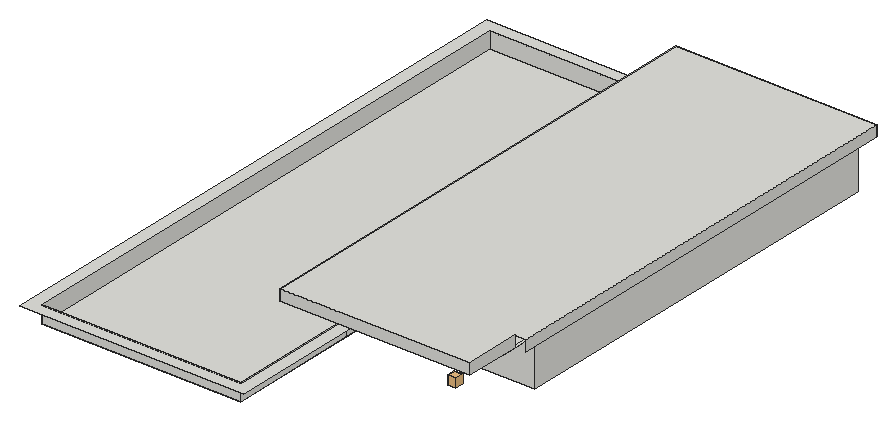
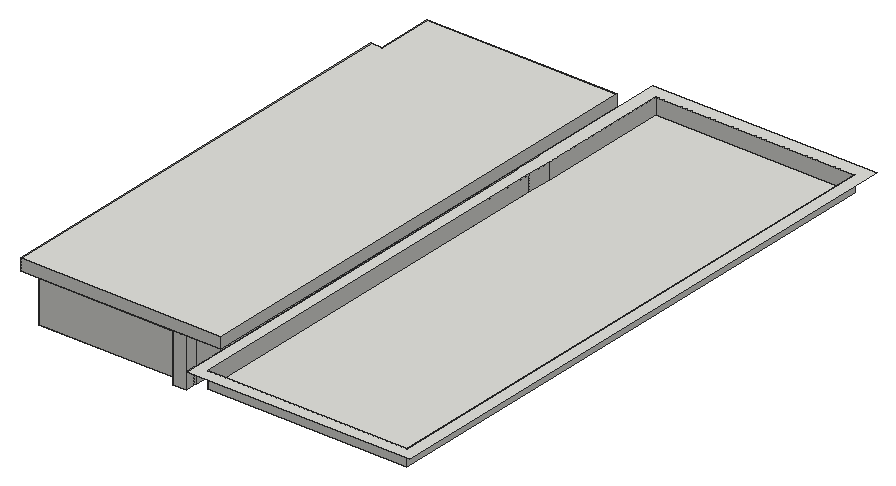
# SketchUp Ruby script. Lengths in inches.
U = 1.inch
M = Sketchup.active_model
def pt(a) = Geom::Point3d.new(a.map { |v| v * U })
def face(e, loops, mat)
  f = e.add_face(loops[0].map { |a| pt(a) })
  loops[1..].each { |l| e.add_face(l.map { |a| pt(a) }).erase! }
  f.material = f.back_material = mat if mat
  f
end
# faces: each face lists its corners as indices into pts; further lists are holes
def faces(e, pts, list, mat = nil) = list.each { |f| face(e, (f[0].is_a?(Array) ? f : [f]).map { |l| l.map { |i| pts[i] } }, mat) }
# xy, xz, yz: faces in a plane at the given z, y or x. An outline is a flat list of corners, or four numbers for a rectangle; further outlines are holes
def ring(l) = l.size == 4 ? [[l[0], l[1]], [l[2], l[1]], [l[2], l[3]], [l[0], l[3]]] : l.each_slice(2).to_a
def flat(e, list, mat, &to3) = list.each { |f| face(e, (f[0].is_a?(Array) ? f : [f]).map { |l| ring(l).map { |u, v| to3.(u, v) } }, mat) }
def xy(e, z, list, mat = nil) = flat(e, list, mat) { |x, y| [x, y, z] }
def xz(e, y, list, mat = nil) = flat(e, list, mat) { |x, z| [x, y, z] }
def yz(e, x, list, mat = nil) = flat(e, list, mat) { |y, z| [x, y, z] }
def lines(e, pts, list) = list.each { |a, b| e.add_line(pt(pts[a]), pt(pts[b])) }
# prism: a flat outline (further loops are holes) pulled along v
def prism(e, loops, v, mat = nil)
  f = face(e, loops, mat); d = Geom::Vector3d.new(v.map { |x| x * U })
  f.pushpull(f.normal.samedirection?(d) ? d.length : -d.length)
end
def box(e, o, s, mat = nil) = prism(e, [[o, [o[0] + s[0], o[1], o[2]], [o[0] + s[0], o[1] + s[1], o[2]], [o[0], o[1] + s[1], o[2]]]], [0, 0, s[2]], mat)
def at(x, y, z, deg = 0) = Geom::Transformation.translation(pt([x, y, z])) * Geom::Transformation.rotation(ORIGIN, Z_AXIS, deg.degrees)
def axes(o, x, y, z) = Geom::Transformation.new([*x, 0, *y, 0, *z, 0, *pt(o).to_a, 1])
def part(name) = M.definitions.add(name)
# library, detail: a bought-in or finely detailed component or shape, given as its bounding box
def library(name, o, s) = part(name).tap { |d| box(d.entities, o, s) }
def detail(e, o, s) = box(e.add_group.entities, o, s)
def put(e, d, t, mat = nil) = e.add_instance(d, t).tap { |i| i.material = mat if mat }
def group(e, t, mat = nil) = e.add_group.tap { |g| g.transformation = t; g.material = mat if mat }.entities
root = M.entities
M.materials.add("Glass_Tinted_Gray").color = [0, 0, 0]
M.materials["Glass_Tinted_Gray"].alpha = 0.125
M.materials.add("[0135_DarkGray]").color = [81, 81, 81]
M.materials.add("[Mirror 02]").color = [229, 229, 229]
M.materials.add("[Terrazzo Light Blue]").color = [196, 214, 227]
M.materials.add("[Wood Veneer 01]").color = [120, 70, 37]
c1 = library("Spot Light",[-5.1,-5.1,-11.05],[10.2,10.2,11.05])
c2 = part("PENTEK_RP Fineline 50S_Sliding_DoorCase_E1")
box(c2.entities,[0,0,0],[1.51,3.66,99.27],"[0135_DarkGray]")
c3 = part("PENTEK_RP Fineline 50S_SlidingDooe_Case_E2")
box(c3.entities,[0,0,0],[96.25,3.66,1.51],"[0135_DarkGray]")
c4 = part("pentek_RP Fineline 50S_SlidingDoor_Case")
put(c4.entities,c2,at(97.76,0,0))
put(c4.entities,c3,at(1.51,0,0))
put(c4.entities,c2,at(0,0,0))
put(c4.entities,c3,at(1.51,0,97.76))
c5 = part("PENTEK_RP Fineline 50S_SlidingDoor_GlazingBead_2")
box(c5.entities,[0,0,0],[0.56,0.59,94.39],"[0135_DarkGray]")
c6 = part("PENTEK_RP Fineline 50S_SlidingDoor_Glass")
box(c6.entities,[0,0,0],[46.58,0.16,94.39],"Glass_Tinted_Gray")
c7 = part("PENTEK_RP Fineline 50S_SlidingDoor_GlazingBead")
box(c7.entities,[0,0,0],[45.47,0.59,0.56],"[0135_DarkGray]")
c8 = part("PENTEK_RP Fineline 50S_SlidingDoor_Leaf_E1")
xy(c8.entities,0,[[0,0,0.93,1.97],[0.93,1.57,1.49,1.97]],"[0135_DarkGray]")
xy(c8.entities,96.25,[[0,0,0.93,0,0.93,1.57,1.49,1.57,1.49,1.97,0,1.97]],"[0135_DarkGray]")
xz(c8.entities,0,[[0,0,0.93,96.25]],"[0135_DarkGray]")
xz(c8.entities,1.57,[[0.93,0,1.49,95.32],[0.93,95.32,1.49,96.25]],"[0135_DarkGray]")
xz(c8.entities,1.97,[[0,0,1.49,96.25]],"[0135_DarkGray]")
yz(c8.entities,0,[[0,0,1.97,96.25]],"[0135_DarkGray]")
yz(c8.entities,0.93,[[0,0,1.57,0.93],[0,0.93,1.57,95.32],[0,95.32,1.57,96.25]],"[0135_DarkGray]")
yz(c8.entities,1.49,[[1.57,0,1.97,95.32],[1.57,95.32,1.97,96.25]],"[0135_DarkGray]")
c9 = part("PENTEK_RP Fineline 50S_SlidingDoor_Leaf_E2")
xy(c9.entities,0,[[0,0,0,1.57,0.56,1.57,0.56,1.97,46.02,1.97,46.02,1.57,46.58,1.57,46.58,0]],"[0135_DarkGray]")
xy(c9.entities,0.93,[[0,0,46.58,1.57]],"[0135_DarkGray]")
xy(c9.entities,1.49,[[0.56,1.57,46.02,1.97]],"[0135_DarkGray]")
xz(c9.entities,0,[[0,0,46.58,0.93]],"[0135_DarkGray]")
xz(c9.entities,1.57,[[0,0,0.56,0.93],[46.02,0,46.58,0.93],[0.56,0.93,46.02,1.49]],"[0135_DarkGray]")
xz(c9.entities,1.97,[[0.56,0,46.02,1.49]],"[0135_DarkGray]")
yz(c9.entities,0,[[0,0,1.57,0.93]],"[0135_DarkGray]")
yz(c9.entities,0.56,[[1.57,0,1.97,0.93],[1.57,0.93,1.97,1.49]],"[0135_DarkGray]")
yz(c9.entities,46.02,[[1.57,0,1.97,0.93],[1.57,0.93,1.97,1.49]],"[0135_DarkGray]")
yz(c9.entities,46.58,[[0,0,1.57,0.93]],"[0135_DarkGray]")
c10 = part("PENTEK_RP Fineline S_SlidingDoor_Leaf1")
put(c10.entities,c5,at(0.93,0,0.93))
put(c10.entities,c5,at(46.96,0,0.93))
put(c10.entities,c6,at(1.49,1.42,0.93))
put(c10.entities,c7,at(1.49,0,0.93))
put(c10.entities,c6,at(1.49,0.59,0.93),"[Terrazzo Light Blue]")
put(c10.entities,c8,at(0,0,0))
put(c10.entities,c8,axes([48.44,0,0],[-1,0,0],[0,1,0],[0,0,1]))
put(c10.entities,c9,axes([0.93,0,96.25],[1,0,0],[0,1,0],[0,0,-1]))
put(c10.entities,c9,at(0.93,0,0))
put(c10.entities,c7,at(1.49,0,94.77))
c11 = part("PENTEK_RP Fineline 50S_SlidingDoor_Leaf2")
put(c11.entities,c6,at(1.49,1.42,0.93))
put(c11.entities,c7,at(1.49,0,94.77))
put(c11.entities,c5,at(46.96,0,0.93))
put(c11.entities,c6,at(1.49,0.59,0.93),"[Mirror 02]")
put(c11.entities,c5,at(0.93,0,0.93))
put(c11.entities,c8,at(0,0,0))
put(c11.entities,c8,axes([48.44,0,0],[-1,0,0],[0,1,0],[0,0,1]))
put(c11.entities,c7,at(1.49,0,0.93))
put(c11.entities,c9,axes([0.93,0,96.25],[1,0,0],[0,1,0],[0,0,-1]))
put(c11.entities,c9,at(0.93,0,0))
c12 = part("PENTEK - Slimmest Steel Sliding Door / Window\#1")
put(c12.entities,c4,at(0,-1.88,-0.09))
put(c12.entities,c10,at(1.51,-2.27,1.42))
put(c12.entities,c11,at(49.32,-0.3,1.42))
c13 = part("Group76\#1")
p = [[0,0,0],[0,0,-13.3125],[-1.22,0,-13.3125],[7.92,-35.18,0],[-7.92,-35.18,0],[7.92,35.18,0],
  [7.92,0,0],[-7.92,35.18,0],[1.22,0,-13.3125],[-7.92,0,0],[0,0,-21.55]]
lines(c13.entities,p,[[0,1],[1,2],[3,4],[5,6],[7,5],[1,8],[9,0],[0,6],[8,10],[4,9],[6,3],[2,10],
  [9,7]])
c14 = part("Rectangle Light\#2")
put(c14.entities,c13,at(0,0,0))
c15 = library("Group\#24",[-0.5,-0.5,0],[156.52,11,0.25])
xy(root,379.1875,[[223.8125,438.06,222.26,438.25,220.8125,438.85,219.5625,439.8,218.61,441.04,218,442.48,217.79,444.03,217.99,445.59,218.58,447.04,219.53,448.28,220.77,449.24,222.22,449.84,223.77,450.06,225.32,449.86,226.77,449.26,228.02,448.3125,228.98,447.08,229.58,445.63,229.79,444.08,229.59,442.52,229,441.08,228.05,439.83,226.81,438.87,225.37,438.27],[274.1875,438.06,272.63,438.25,271.1875,438.85,269.9375,439.8,268.98,441.04,268.375,442.48,268.17,444.03,268.36,445.59,268.96,447.04,269.91,448.28,271.15,449.24,272.59,449.84,274.14,450.06,275.7,449.86,277.15,449.26,278.39,448.3125,279.35,447.08,279.96,445.63,280.17,444.08,279.97,442.52,279.375,441.08,278.42,439.83,277.19,438.87,275.74,438.27],[322.8125,438.06,321.26,438.25,319.8125,438.85,318.5625,439.8,317.61,441.04,317,442.48,316.79,444.03,316.99,445.59,317.58,447.04,318.53,448.28,319.77,449.24,321.22,449.84,322.77,450.06,324.32,449.86,325.77,449.26,327.02,448.3125,327.98,447.08,328.58,445.63,328.79,444.08,328.59,442.52,328,441.08,327.05,439.83,325.81,438.87,324.37,438.27],[388.8125,438.06,387.26,438.25,385.8125,438.85,384.5625,439.8,383.61,441.04,383,442.48,382.79,444.03,382.99,445.59,383.58,447.04,384.53,448.28,385.77,449.24,387.22,449.84,388.77,450.06,390.32,449.86,391.77,449.26,393.02,448.3125,393.98,447.08,394.58,445.63,394.79,444.08,394.59,442.52,394,441.08,393.05,439.83,391.81,438.87,390.37,438.27],[223.79,540.64,222.24,540.85,220.79,541.45,219.55,542.4,218.59,543.64,217.99,545.09,217.79,546.64,217.99,548.2,218.59,549.64,219.55,550.89,220.79,551.84,222.24,552.4375,223.79,552.64,225.34,552.4375,226.79,551.84,228.03,550.89,228.99,549.64,229.59,548.2,229.79,546.64,229.59,545.09,228.99,543.64,228.03,542.4,226.79,541.45,225.34,540.85],
  [274.17,540.64,272.61,540.85,271.17,541.45,269.92,542.4,268.97,543.64,268.37,545.09,268.17,546.64,268.37,548.2,268.97,549.64,269.92,550.89,271.17,551.84,272.61,552.4375,274.17,552.64,275.72,552.4375,277.17,551.84,278.41,550.89,279.36,549.64,279.96,548.2,280.17,546.64,279.96,545.09,279.36,543.64,278.41,542.4,277.17,541.45,275.72,540.85],[322.79,540.64,321.24,540.85,319.79,541.45,318.55,542.4,317.59,543.64,316.99,545.09,316.79,546.64,316.99,548.2,317.59,549.64,318.55,550.89,319.79,551.84,321.24,552.4375,322.79,552.64,324.34,552.4375,325.79,551.84,327.03,550.89,327.99,549.64,328.59,548.2,328.79,546.64,328.59,545.09,327.99,543.64,327.03,542.4,325.79,541.45,324.34,540.85],[388.79,540.64,387.24,540.85,385.79,541.45,384.55,542.4,383.59,543.64,382.99,545.09,382.79,546.64,382.99,548.2,383.59,549.64,384.55,550.89,385.79,551.84,387.24,552.4375,388.79,552.64,390.34,552.4375,391.79,551.84,393.03,550.89,393.99,549.64,394.59,548.2,394.79,546.64,394.59,545.09,393.99,543.64,393.03,542.4,391.79,541.45,390.34,540.85]])
xy(root,381.03,[[572.68,554.8125,578.99,562.125]])
xy(root,384,[[192.6,398.16,438.02,1088.46],[452.87,593.61,469.06,1087.125],[469.06,593.61,469.08,1091.4],[469.08,593.61,644.41,1091.4],[452.87,1087.125,469.06,1091.4],
  [452.87,1091.4,469.06,1103.3125]])
xy(root,404.125,[[[177.75,383.3125,452.87,1103.3125],[192.6,398.16,438.02,1088.46]]])
xy(root,408.9,[[484.27,562.125,554.02,593.61]])
xy(root,429.22,[[484.27,562.125,554.02,593.61]])
xy(root,431.7,[[597.99,562.125,631.02,589.625]])
xy(root,444,[[452.87,562.125,469.06,593.61],[469.06,562.125,641.5625,593.61],[641.5625,562.125,644.41,593.61],[452.87,593.61,469.06,1087.125],[469.06,593.61,641.5625,1087.125],
  [641.5625,593.61,644.41,1087.125],[452.87,1087.125,469.06,1103.3125],[469.06,1087.125,644.41,1091.4],[644.41,1087.125,657.75,1103.3125],[469.06,1091.4,644.41,1103.3125]])
xy(root,444,[[[410.81,492.5,410.81,1103.3125,452.87,1103.3125,452.87,562.125,644.41,562.125,644.41,492.5],[577.39,512.37,578.68,512.54,579.89,513.04,580.93,513.84,581.72,514.87,582.22,516.08,582.39,517.37,582.22,518.67,581.72,519.87,580.93,520.91,579.89,521.7,578.68,522.2,577.39,522.37,576.1,522.2,574.89,521.7,573.86,520.91,573.06,519.87,572.5625,518.67,572.39,517.37,572.5625,516.08,573.06,514.87,573.86,513.84,574.89,513.04,576.1,512.54],[470.07,512.37,471.37,512.54,472.57,513.04,473.61,513.84,474.4,514.87,474.9,516.08,475.07,517.37,474.9,518.67,474.4,519.87,473.61,520.91,472.57,521.7,471.37,522.2,470.07,522.37,468.78,522.2,467.57,521.7,466.54,520.91,465.74,519.87,465.24,518.67,465.07,517.37,465.24,516.08,465.74,514.87,466.54,513.84,467.57,513.04,468.78,512.54],[527.61,513.44,528.625,513.57,529.58,513.96,530.39,514.59,531.02,515.4,531.41,516.35,531.54,517.37,531.41,518.39,531.02,519.34,530.39,520.16,529.58,520.78,528.625,521.18,527.61,521.31,526.59,521.18,525.64,520.78,524.82,520.16,524.2,519.34,523.8,518.39,523.67,517.37,523.8,516.35,524.2,515.4,524.82,514.59,525.64,513.96,526.59,513.57],[616.93,513.71,617.88,513.83,618.76,514.2,619.52,514.78,620.1,515.54,620.47,516.42,620.59,517.37,620.47,518.32,620.1,519.2,619.52,519.96,618.76,520.55,617.88,520.91,616.93,521.04,615.98,520.91,615.1,520.55,614.34,519.96,613.76,519.2,613.39,518.32,613.27,517.37,613.39,516.42,613.76,515.54,614.34,514.78,615.1,514.2,615.98,513.83]]],"[Wood Veneer 01]")
xy(root,457.625,[[410.81,492.5,644.41,492.5,644.41,562.125,657.75,562.125,657.75,1103.3125,410.81,1103.3125]])
xz(root,398.16,[[192.6,384,438.02,404.125]])
xz(root,492.5,[[410.81,444,644.41,457.625]])
xz(root,593.61,[[452.87,384,469.06,444],[[469.06,384,644.41,444],[484.27,408.9,554.02,429.22]]])
xz(root,1087.125,[[452.87,384,469.06,444]])
xz(root,1088.46,[[192.6,384,438.02,404.125]])
xz(root,1091.4,[[469.06,384,644.41,444]])
xz(root,1103.3125,[[452.87,384,469.06,444],[410.81,444,657.75,457.625]])
yz(root,192.6,[[398.16,384,1088.46,404.125]])
yz(root,410.81,[[492.5,444,1103.3125,457.625]])
yz(root,438.02,[[398.16,384,562.125,404.125],[562.125,384,593.61,404.125],[593.61,384,1087.125,404.125],[1087.125,384,1088.46,404.125]])
yz(root,452.87,[[593.61,384,1087.125,404.125],[1087.125,384,1091.4,404.125],[1091.4,384,1103.3125,404.125],[562.125,404.125,593.61,444],[593.61,404.125,1087.125,444],
  [1087.125,404.125,1103.3125,444]])
yz(root,469.06,[[593.61,384,1087.125,444],[1087.125,384,1091.4,444],[1091.4,384,1103.3125,444]])
yz(root,484.27,[[562.125,408.9,593.61,429.22]])
yz(root,554.02,[[562.125,408.9,593.61,429.22]])
yz(root,644.41,[[593.61,384,1091.4,444],[492.5,444,562.125,457.625]])
yz(root,657.75,[[562.125,444,1103.3125,457.625]])
p = [[470.07,512.37,444],[468.78,512.54,444],[468.78,512.54,445.375],[470.07,512.37,445.375],[471.37,512.54,444],[471.37,512.54,445.375],
  [577.39,512.37,444],[576.1,512.54,444],[576.1,512.54,445.375],[577.39,512.37,445.375],[578.68,512.54,444],[578.68,512.54,445.375],
  [467.57,513.04,444],[467.57,513.04,445.375],[472.57,513.04,444],[472.57,513.04,445.375],[574.89,513.04,444],[574.89,513.04,445.375],
  [579.89,513.04,444],[579.89,513.04,445.375],[466.54,513.84,444],[466.54,513.84,445.375],[473.61,513.84,444],[473.61,513.84,445.375],
  [573.86,513.84,444],[573.86,513.84,445.375],[580.93,513.84,444],[580.93,513.84,445.375],[527.61,513.44,444],[526.59,513.57,444],
  [526.59,513.57,445.375],[527.61,513.44,445.375],[528.625,513.57,444],[528.625,513.57,445.375],[525.64,513.96,444],[525.64,513.96,445.375],
  [529.58,513.96,444],[529.58,513.96,445.375],[616.93,513.71,444],[615.98,513.83,444],[615.98,513.83,445.625],[616.93,513.71,445.625],
  [617.88,513.83,444],[617.88,513.83,445.625],[465.74,514.87,444],[465.74,514.87,445.375],[474.4,514.87,444],[474.4,514.87,445.375],
  [573.06,514.87,444],[573.06,514.87,445.375],[581.72,514.87,444],[581.72,514.87,445.375],[615.1,514.2,444],[615.1,514.2,445.625],
  [618.76,514.2,444],[618.76,514.2,445.625],[524.82,514.59,444],[524.82,514.59,445.375],[530.39,514.59,444],[530.39,514.59,445.375],
  [614.34,514.78,444],[614.34,514.78,445.625],[619.52,514.78,444],[619.52,514.78,445.625],[524.2,515.4,444],[524.2,515.4,445.375],
  [531.02,515.4,444],[531.02,515.4,445.375],[613.76,515.54,444],[613.76,515.54,445.625],[620.1,515.54,444],[620.1,515.54,445.625],
  [465.24,516.08,444],[465.24,516.08,445.375],[474.9,516.08,444],[474.9,516.08,445.375],[572.5625,516.08,444],[572.5625,516.08,445.375],
  [582.22,516.08,444],[582.22,516.08,445.375],[523.8,516.35,444],[523.8,516.35,445.375],[531.41,516.35,444],[531.41,516.35,445.375],
  [613.39,516.42,444],[613.39,516.42,445.625],[620.47,516.42,444],[620.47,516.42,445.625],[465.07,517.37,444],[465.07,517.37,445.375],
  [475.07,517.37,444],[475.07,517.37,445.375],[572.39,517.37,444],[572.39,517.37,445.375],[582.39,517.37,444],[582.39,517.37,445.375],
  [523.67,517.37,444],[523.67,517.37,445.375],[531.54,517.37,444],[531.54,517.37,445.375],[613.27,517.37,444],[613.27,517.37,445.625],
  [620.59,517.37,444],[620.59,517.37,445.625],[465.24,518.67,444],[465.24,518.67,445.375],[474.9,518.67,444],[474.9,518.67,445.375],
  [523.8,518.39,444],[523.8,518.39,445.375],[531.41,518.39,444],[531.41,518.39,445.375],[572.5625,518.67,444],[572.5625,518.67,445.375],
  [582.22,518.67,444],[582.22,518.67,445.375],[613.39,518.32,444],[613.39,518.32,445.625],[620.47,518.32,444],[620.47,518.32,445.625],
  [613.76,519.2,444],[613.76,519.2,445.625],[620.1,519.2,444],[620.1,519.2,445.625],[524.2,519.34,444],[524.2,519.34,445.375],
  [531.02,519.34,444],[531.02,519.34,445.375],[465.74,519.87,444],[465.74,519.87,445.375],[474.4,519.87,444],[474.4,519.87,445.375],
  [573.06,519.87,444],[573.06,519.87,445.375],[581.72,519.87,444],[581.72,519.87,445.375],[614.34,519.96,444],[614.34,519.96,445.625],
  [619.52,519.96,444],[619.52,519.96,445.625],[524.82,520.16,444],[524.82,520.16,445.375],[530.39,520.16,444],[530.39,520.16,445.375],
  [466.54,520.91,444],[466.54,520.91,445.375],[473.61,520.91,444],[473.61,520.91,445.375],[573.86,520.91,444],[573.86,520.91,445.375],
  [580.93,520.91,444],[580.93,520.91,445.375],[615.1,520.55,444],[615.1,520.55,445.625],[618.76,520.55,444],[618.76,520.55,445.625],
  [525.64,520.78,444],[525.64,520.78,445.375],[529.58,520.78,444],[529.58,520.78,445.375],[615.98,520.91,444],[615.98,520.91,445.625],
  [617.88,520.91,444],[617.88,520.91,445.625],[526.59,521.18,444],[526.59,521.18,445.375],[528.625,521.18,444],[528.625,521.18,445.375],
  [467.57,521.7,444],[467.57,521.7,445.375],[472.57,521.7,444],[472.57,521.7,445.375],[574.89,521.7,444],[574.89,521.7,445.375],
  [579.89,521.7,444],[579.89,521.7,445.375],[616.93,521.04,444],[616.93,521.04,445.625],[527.61,521.31,444],[527.61,521.31,445.375],
  [468.78,522.2,444],[468.78,522.2,445.375],[471.37,522.2,444],[471.37,522.2,445.375],[576.1,522.2,444],[576.1,522.2,445.375],
  [578.68,522.2,444],[578.68,522.2,445.375],[470.07,522.37,444],[470.07,522.37,445.375],[577.39,522.37,444],[577.39,522.37,445.375],
  [469.06,562.125,384],[469.06,593.61,384]]
faces(root,p,[[0,1,2,3],[4,0,3,5],[6,7,8,9],[10,6,9,11],[1,12,13,2],[14,4,5,15],[7,16,17,8],[18,10,11,19],
  [12,20,21,13],[22,14,15,23],[16,24,25,17],[26,18,19,27],[28,29,30,31],[32,28,31,33],[29,34,35,30],[36,32,33,37],
  [38,39,40,41],[42,38,41,43],[20,44,45,21],[46,22,23,47],[24,48,49,25],[50,26,27,51],[39,52,53,40],[54,42,43,55],
  [34,56,57,35],[58,36,37,59],[52,60,61,53],[62,54,55,63],[56,64,65,57],[66,58,59,67],[60,68,69,61],[70,62,63,71],
  [44,72,73,45],[74,46,47,75],[48,76,77,49],[78,50,51,79],[64,80,81,65],[82,66,67,83],[68,84,85,69],[86,70,71,87],
  [72,88,89,73],[90,74,75,91],[76,92,93,77],[94,78,79,95],[80,96,97,81],[98,82,83,99],[84,100,101,85],[102,86,87,103],
  [88,104,105,89],[106,90,91,107],[96,108,109,97],[110,98,99,111],[92,112,113,93],[114,94,95,115],[100,116,117,101],[118,102,103,119],
  [116,120,121,117],[122,118,119,123],[108,124,125,109],[126,110,111,127],[104,128,129,105],[130,106,107,131],[112,132,133,113],[134,114,115,135],
  [120,136,137,121],[138,122,123,139],[124,140,141,125],[142,126,127,143],[128,144,145,129],[146,130,131,147],[132,148,149,133],[150,134,135,151],
  [136,152,153,137],[154,138,139,155],[140,156,157,141],[158,142,143,159],[152,160,161,153],[162,154,155,163],[156,164,165,157],[166,158,159,167],
  [144,168,169,145],[170,146,147,171],[148,172,173,149],[174,150,151,175],[160,176,177,161],[176,162,163,177],[164,178,179,165],[178,166,167,179],
  [168,180,181,169],[182,170,171,183],[172,184,185,173],[186,174,175,187],[180,188,189,181],[188,182,183,189],[184,190,191,185],[190,186,187,191]])
lines(root,p,[[192,193]])
g1 = group(root,at(294.91,832.72,380.0625))
xy(g1,0,[[6,0,4.45,0.2,3,0.8,1.76,1.76,0.8,3,0.2,4.45,0,6,0.2,7.55,0.8,9,1.76,10.24,3,11.2,4.45,11.8,6,12,7.55,11.8,9,11.2,10.24,10.24,11.2,9,11.8,7.55,12,6,11.8,4.45,11.2,3,10.24,1.76,9,0.8,7.55,0.2],[6,59.5625,4.45,59.77,3,60.37,1.76,61.32,0.8,62.5625,0.2,64.01,0,65.5625,0.2,67.12,0.8,68.5625,1.76,69.81,3,70.76,4.45,71.36,6,71.5625,7.55,71.36,9,70.76,10.24,69.81,11.2,68.5625,11.8,67.12,12,65.5625,11.8,64.01,11.2,62.5625,10.24,61.32,9,60.37,7.55,59.77],[6,176.8125,4.45,177.02,3,177.62,1.76,178.57,0.8,179.8125,0.2,181.26,0,182.8125,0.2,184.37,0.8,185.8125,1.76,187.06,3,188.01,4.45,188.61,6,188.8125,7.55,188.61,9,188.01,10.24,187.06,11.2,185.8125,11.8,184.37,12,182.8125,11.8,181.26,11.2,179.8125,10.24,178.57,9,177.62,7.55,177.02]])
g2 = group(root,at(503.16,768.54,380.125))
xy(g2,0,[[6,0,4.45,0.2,3,0.8,1.76,1.76,0.8,3,0.2,4.45,0,6,0.2,7.55,0.8,9,1.76,10.24,3,11.2,4.45,11.8,6,12,7.55,11.8,9,11.2,10.24,10.24,11.2,9,11.8,7.55,12,6,11.8,4.45,11.2,3,10.24,1.76,9,0.8,7.55,0.2],[14.44,107.125,12.89,107.33,11.44,107.93,10.2,108.88,9.25,110.125,8.65,111.57,8.44,113.125,8.65,114.68,9.25,116.125,10.2,117.37,11.44,118.32,12.89,118.92,14.44,119.125,15.99,118.92,17.44,118.32,18.68,117.37,19.64,116.125,20.24,114.68,20.44,113.125,20.24,111.57,19.64,110.125,18.68,108.88,17.44,107.93,15.99,107.33]])
put(root,c1,axes([575.75,556.15,381.63],[-1,0,0],[0,1,0],[0,0,-1]))
put(root,c12,axes([484.89,562.58,408.92],[0.69642,0,0],[0,0.2,0],[0,0,0.20461]))
put(root,c14,at(496.99,669.47,443.99))
put(root,c15,at(465.07,512.37,445.375))
